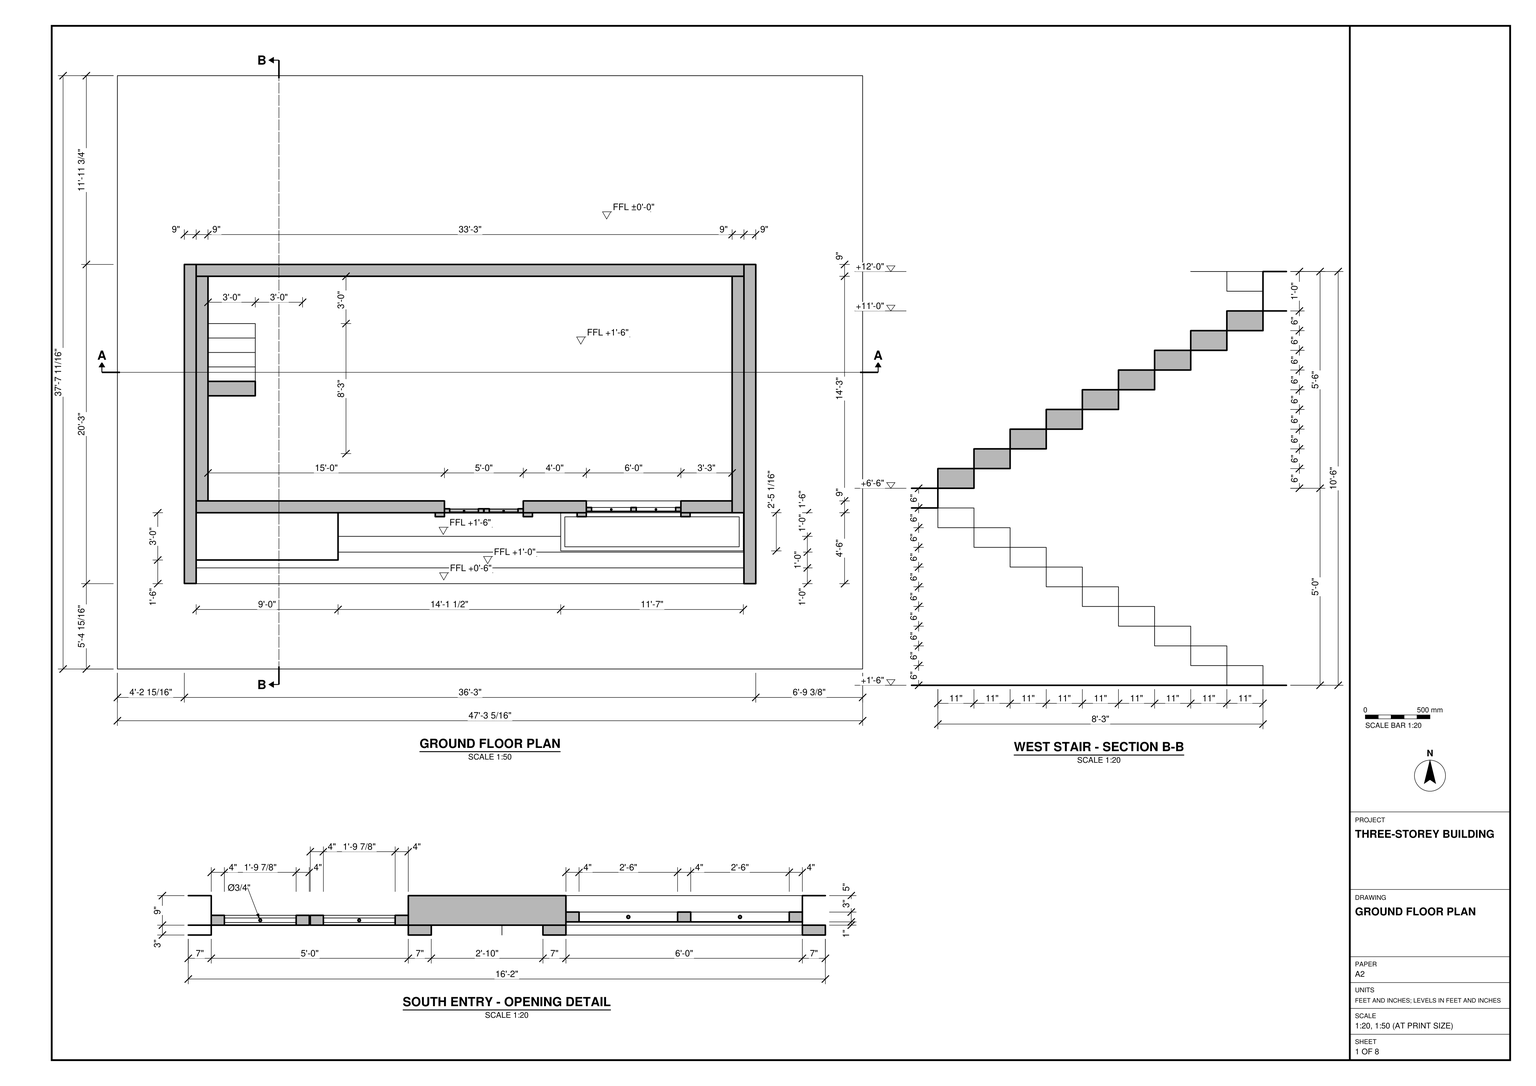
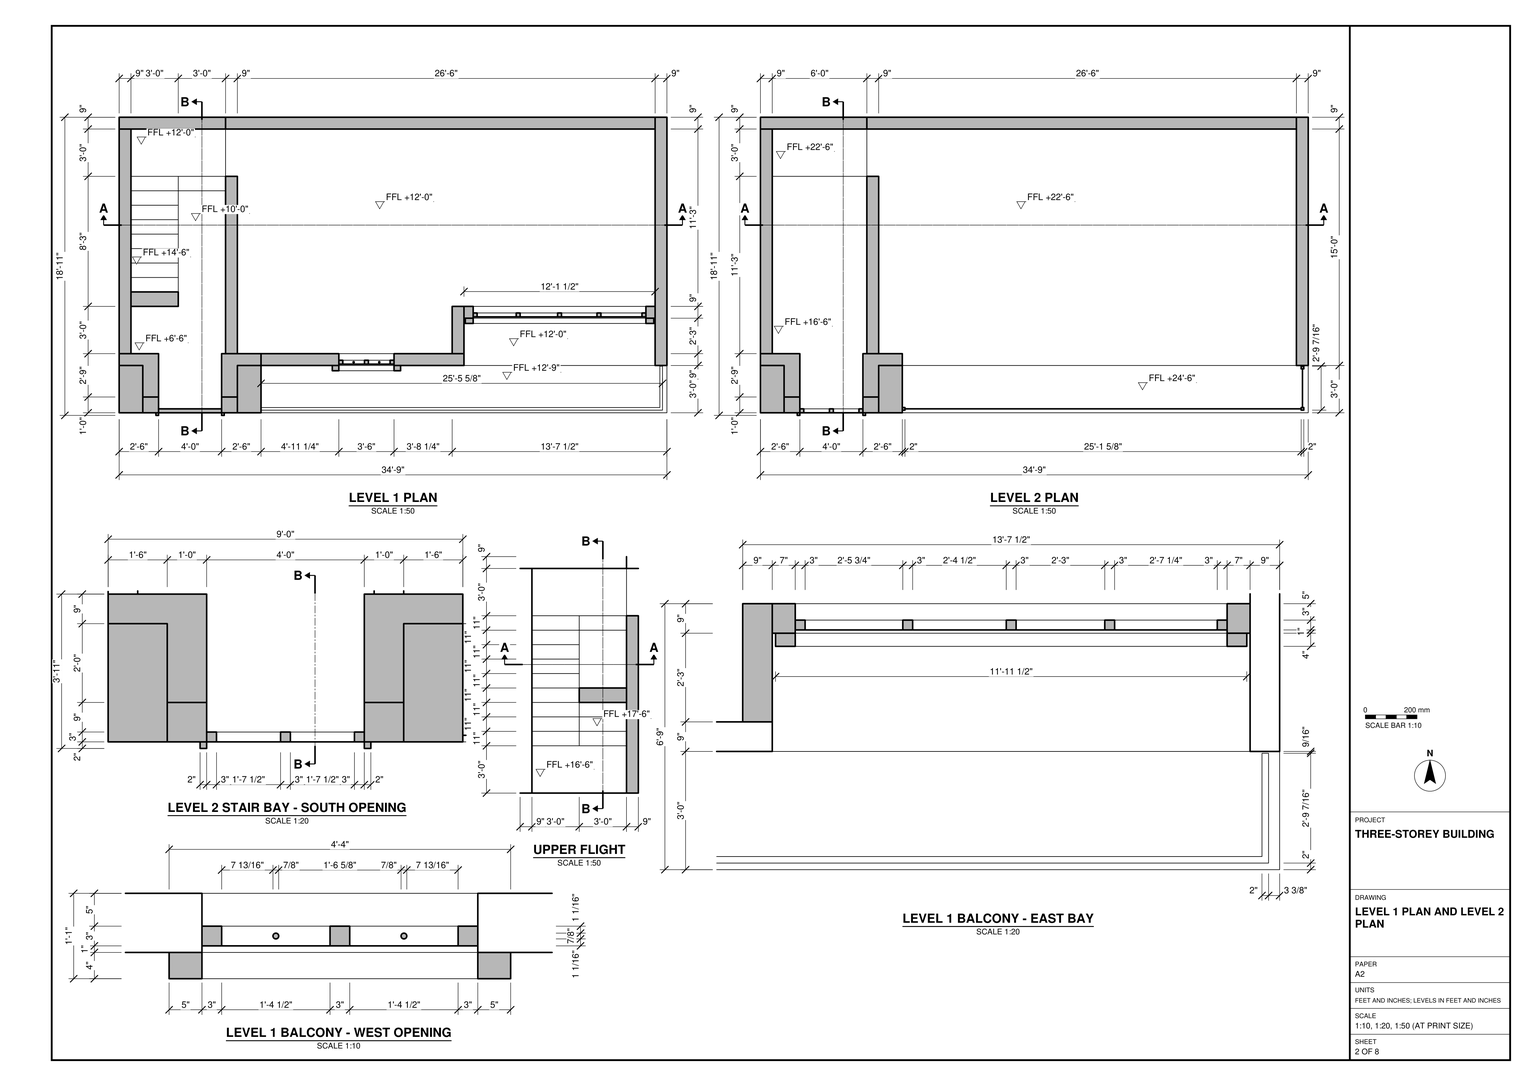
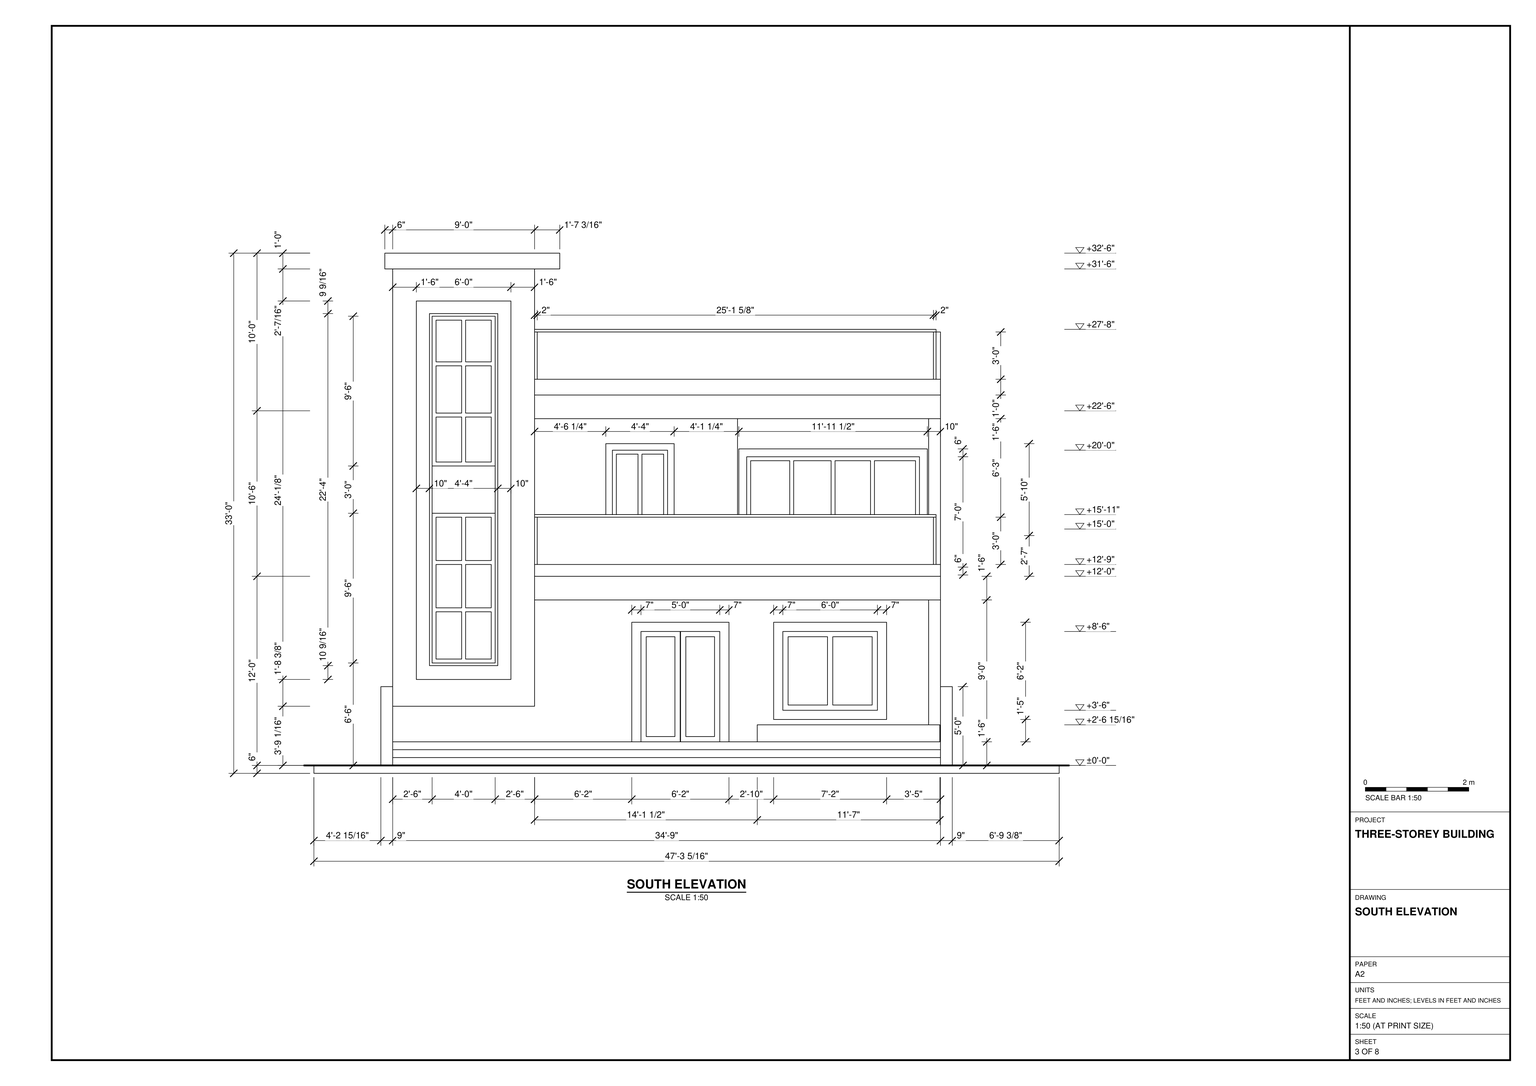
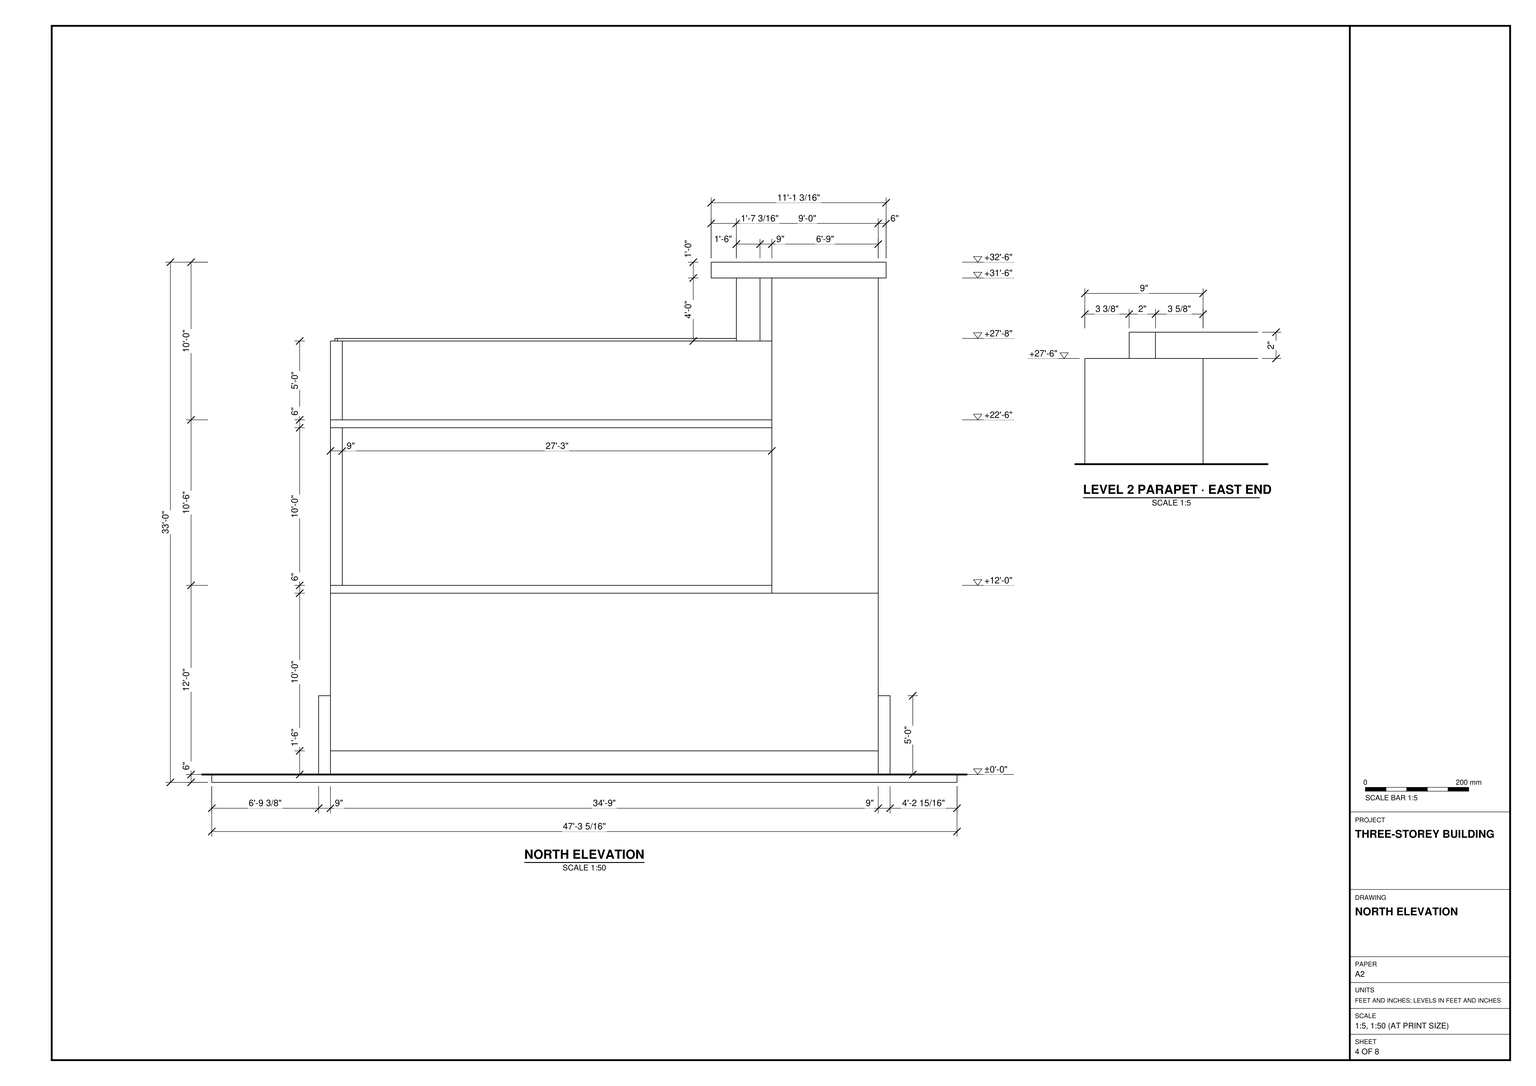
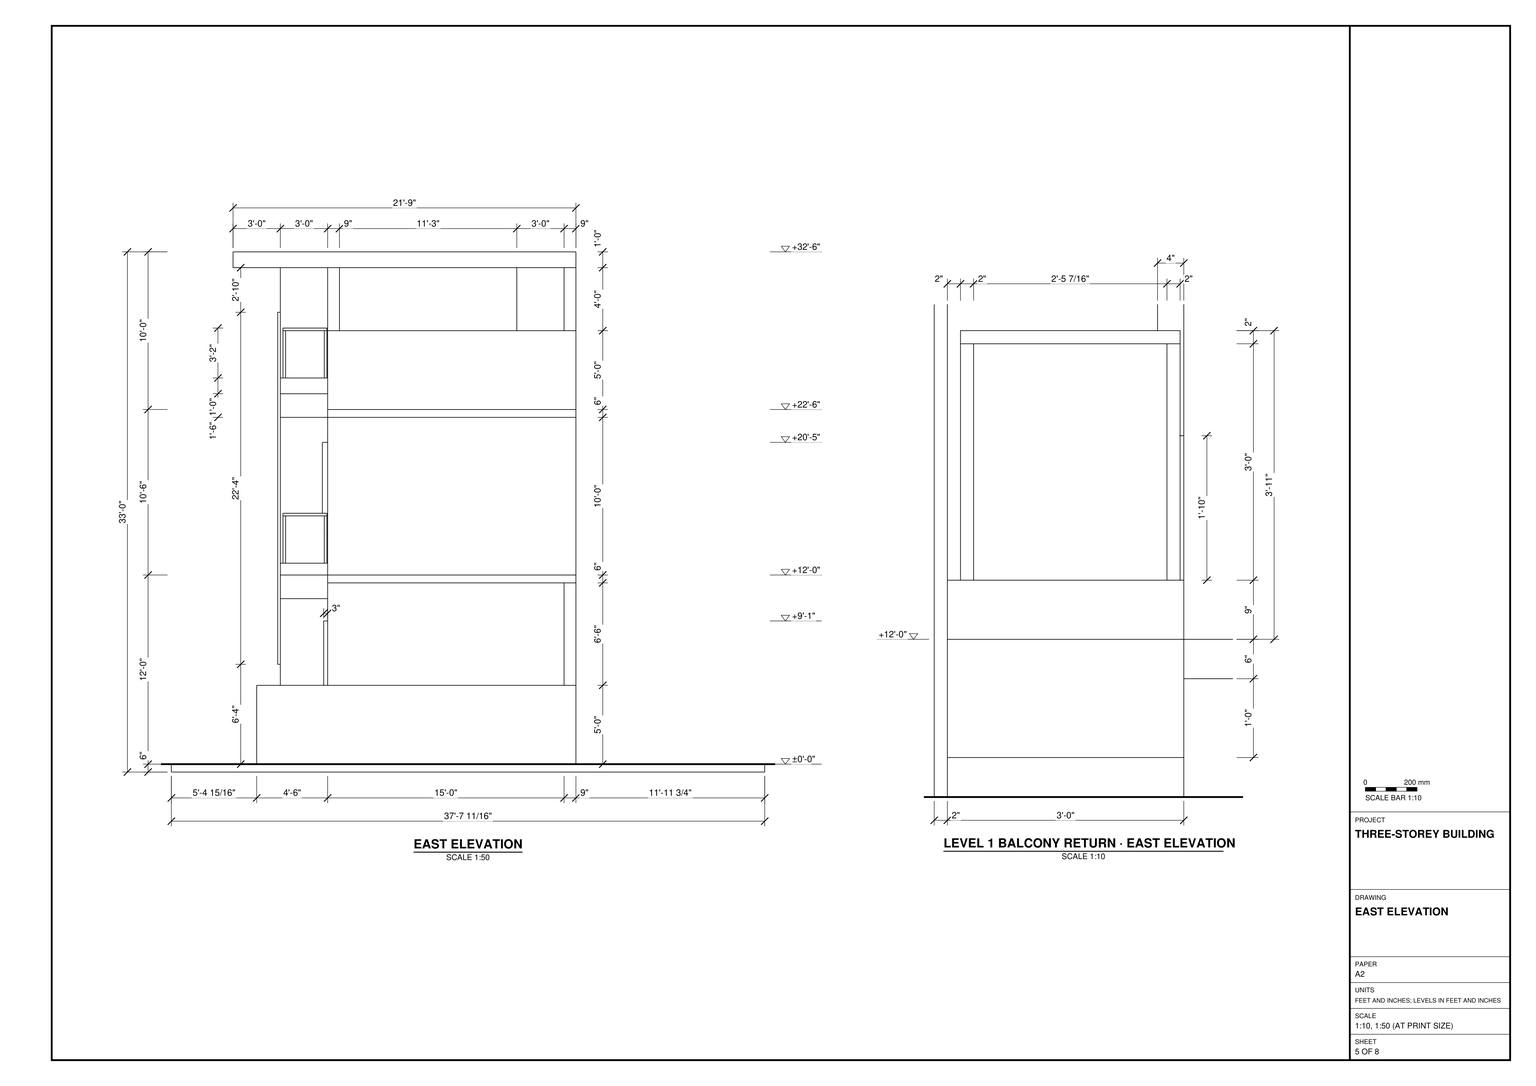
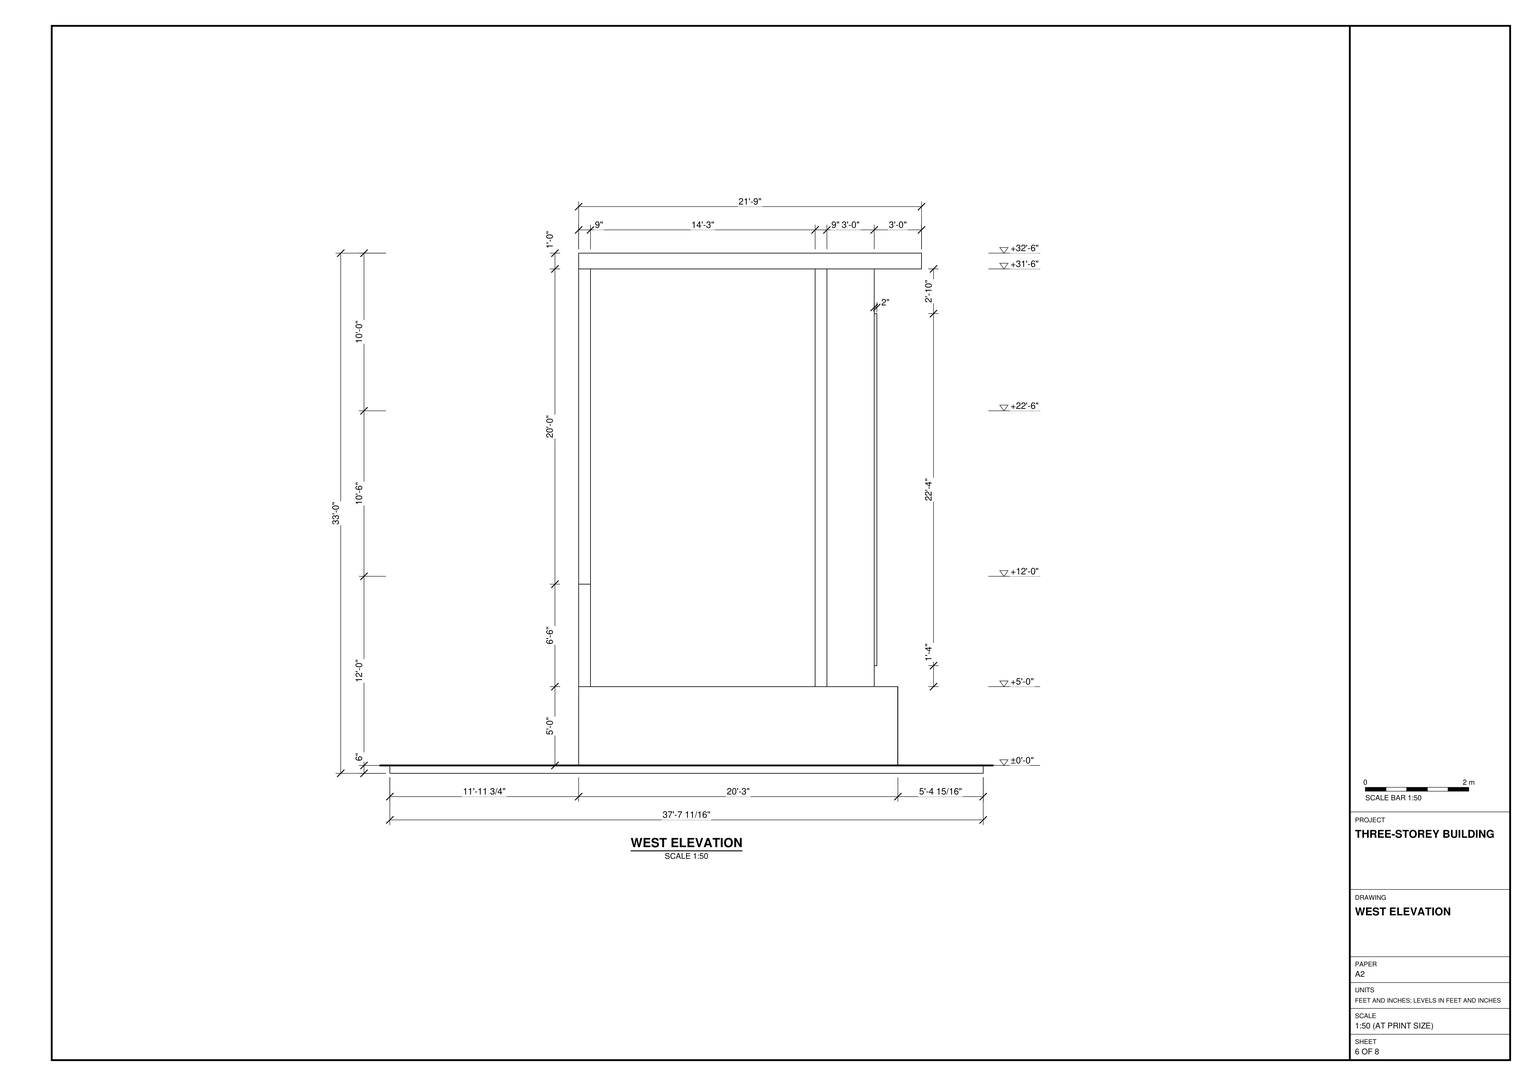
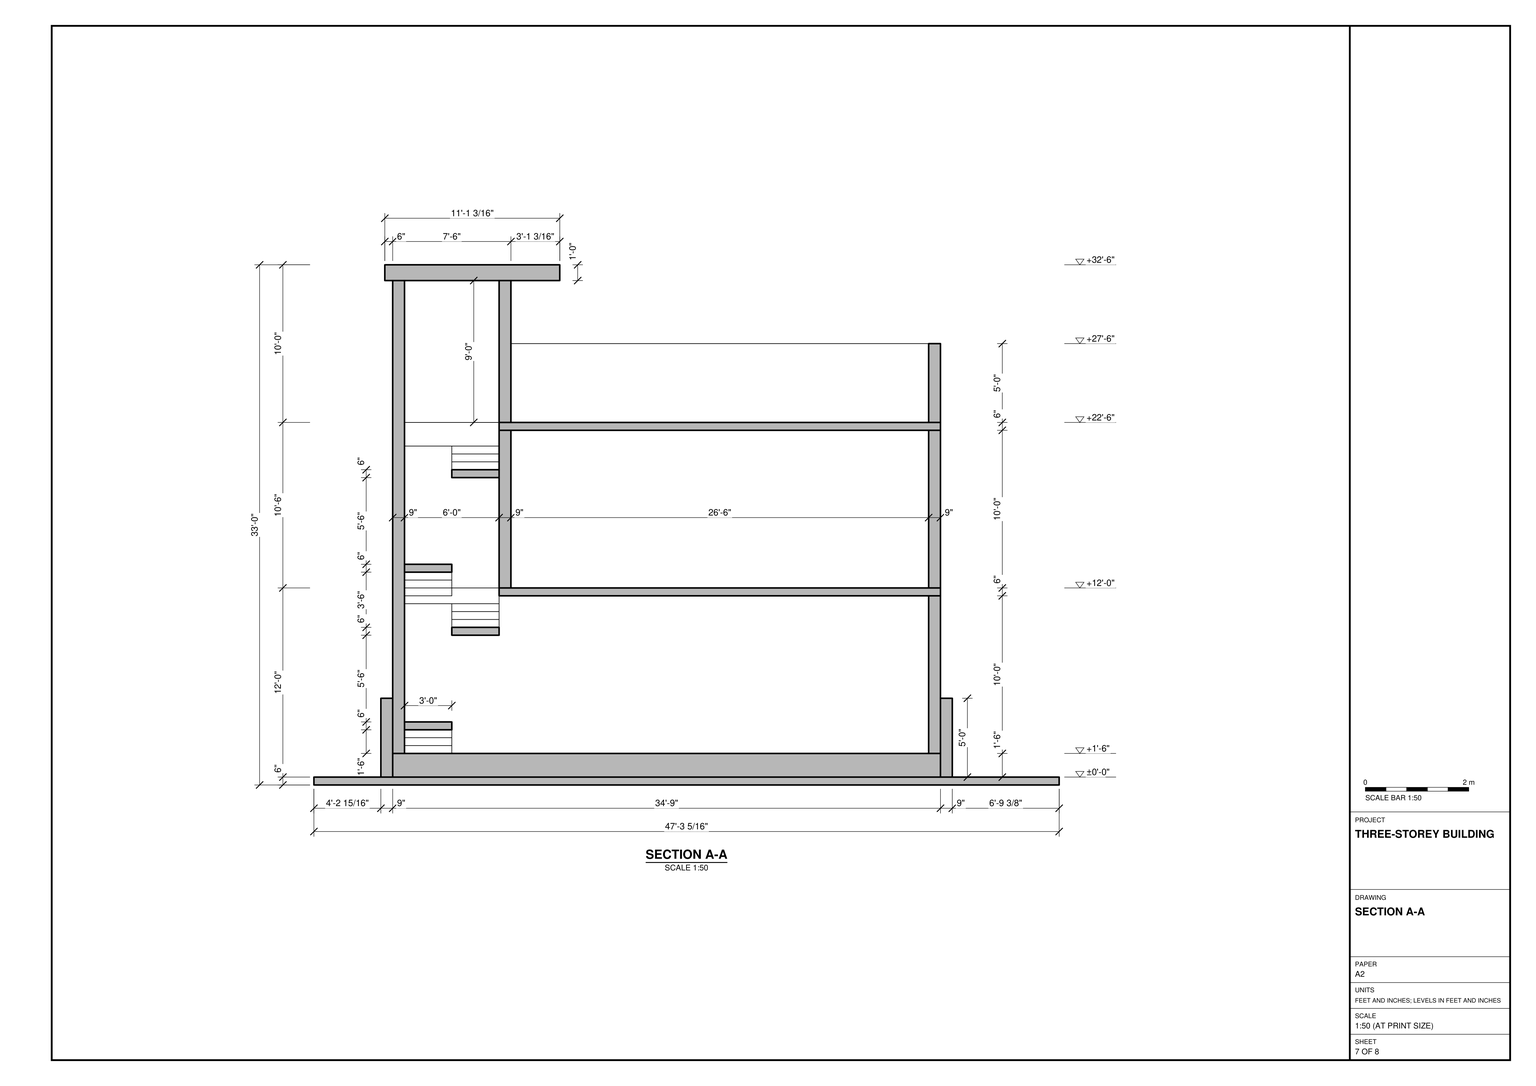
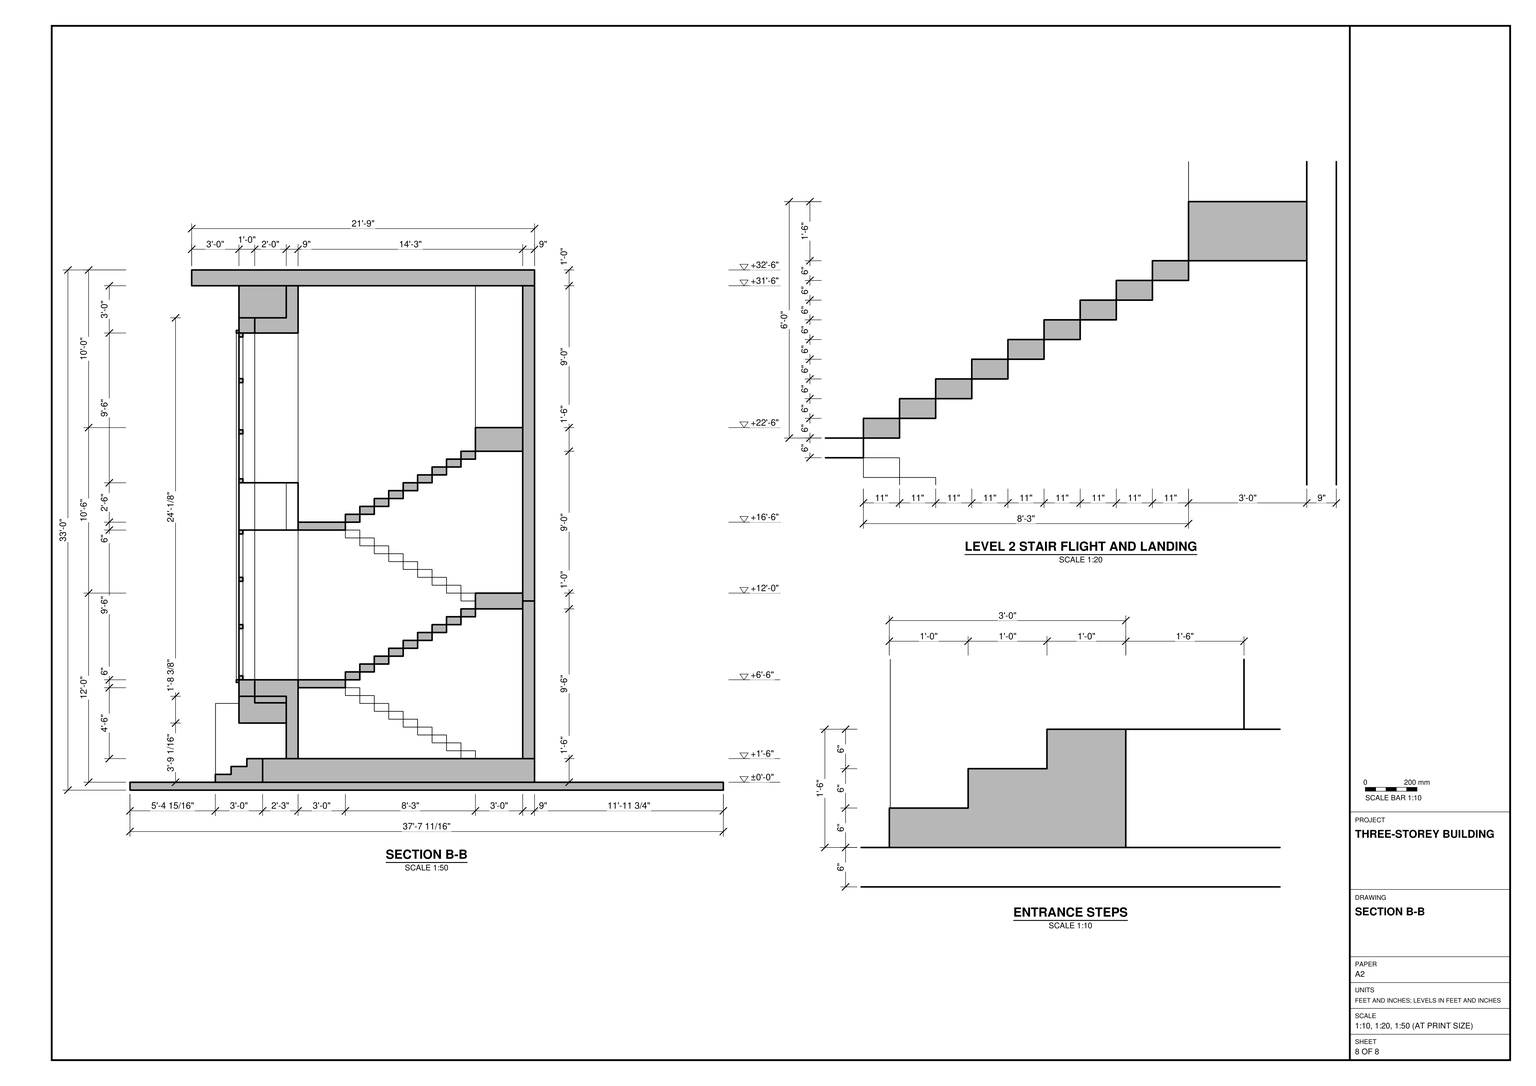
Build the three-storey building and its rectangular site base in SketchUp from task_files/diagram_01.pdf. Work in feet and inches. Including the base, the model measures 47'-3 5/16" east to west, 37'-7 11/16" north to south and 33'-0" from bottom to top. Use ±0'-0" as the ground datum, +12'-0" for Level 1 and +22'-6" for Level 2.

Locate the building on the base using the setbacks on the ground floor plan. Model the floor slabs, walls at their drawn thicknesses, and the south steps leading to the raised entry at +1'-6". Fit the paired entry door and the window to its east with the frames and pane divisions shown. At the west end, build the stair flights, intermediate landings and slab openings together so the stair connects the levels. Match the stacked glazing and projecting flat cap of the stair tower to the south elevation. Form the Level 1 balcony with its recessed east bay, and carry the upper terrace guard across the south side as drawn.

Keep shell elements such as walls, slabs and roof, and each furniture or joinery piece shown, in separate groups or components. Use components for repeated parts. Decor and loose items may be any suitable library components. Save one SketchUp model as output_files/three_storey_building_with_a_west_stair_tower.skp.

# SketchUp Ruby script. Lengths in inches.
U = 1.inch
M = Sketchup.active_model
def pt(a) = Geom::Point3d.new(a.map { |v| v * U })
def face(e, loops, mat)
  f = e.add_face(loops[0].map { |a| pt(a) })
  loops[1..].each { |l| e.add_face(l.map { |a| pt(a) }).erase! }
  f.material = f.back_material = mat if mat
  f
end
# faces: each face lists its corners as indices into pts; further lists are holes
def faces(e, pts, list, mat = nil) = list.each { |f| face(e, (f[0].is_a?(Array) ? f : [f]).map { |l| l.map { |i| pts[i] } }, mat) }
# xy, xz, yz: faces in a plane at the given z, y or x. An outline is a flat list of corners, or four numbers for a rectangle; further outlines are holes
def ring(l) = l.size == 4 ? [[l[0], l[1]], [l[2], l[1]], [l[2], l[3]], [l[0], l[3]]] : l.each_slice(2).to_a
def flat(e, list, mat, &to3) = list.each { |f| face(e, (f[0].is_a?(Array) ? f : [f]).map { |l| ring(l).map { |u, v| to3.(u, v) } }, mat) }
def xy(e, z, list, mat = nil) = flat(e, list, mat) { |x, y| [x, y, z] }
def xz(e, y, list, mat = nil) = flat(e, list, mat) { |x, z| [x, y, z] }
def yz(e, x, list, mat = nil) = flat(e, list, mat) { |y, z| [x, y, z] }
def lines(e, pts, list) = list.each { |a, b| e.add_line(pt(pts[a]), pt(pts[b])) }
# prism: a flat outline (further loops are holes) pulled along v
def prism(e, loops, v, mat = nil)
  f = face(e, loops, mat); d = Geom::Vector3d.new(v.map { |x| x * U })
  f.pushpull(f.normal.samedirection?(d) ? d.length : -d.length)
end
def box(e, o, s, mat = nil) = prism(e, [[o, [o[0] + s[0], o[1], o[2]], [o[0] + s[0], o[1] + s[1], o[2]], [o[0], o[1] + s[1], o[2]]]], [0, 0, s[2]], mat)
def at(x, y, z, deg = 0) = Geom::Transformation.translation(pt([x, y, z])) * Geom::Transformation.rotation(ORIGIN, Z_AXIS, deg.degrees)
def axes(o, x, y, z) = Geom::Transformation.new([*x, 0, *y, 0, *z, 0, *pt(o).to_a, 1])
def part(name) = M.definitions.add(name)
# library, detail: a bought-in or finely detailed component or shape, given as its bounding box
def library(name, o, s) = part(name).tap { |d| box(d.entities, o, s) }
def detail(e, o, s) = box(e.add_group.entities, o, s)
def put(e, d, t, mat = nil) = e.add_instance(d, t).tap { |i| i.material = mat if mat }
def group(e, t, mat = nil) = e.add_group.tap { |g| g.transformation = t; g.material = mat if mat }.entities
root = M.entities
M.materials.add("[Color M05]").color = [114, 114, 114]
M.materials.add("[Color M06]").color = [86, 86, 86]
M.materials.add("[Color M07]").color = [58, 58, 58]
M.materials.add("[Color M09]").color = [0, 0, 0]
M.materials.add("[Grass Dark Green]").color = [106, 157, 55]
M.materials.add("[Translucent Glass Gray]").color = [128, 128, 128]
M.materials["[Translucent Glass Gray]"].alpha = 0.5
M.materials.add("[Wood Veneer 01]").color = [120, 70, 37]
c1 = part("Group\#8")
prism(c1.entities,[[[0,0.2,0.2],[0,0.09,0.34],[0,0.02,0.51],[0,0,0.6875],[0,0.02,0.87],[0,0.09,1.03],[0,0.2,1.17],[0,0.34,1.28],[0,0.51,1.35],[0,0.6875,1.375],[0,0.87,1.35],[0,1.03,1.28],[0,1.17,1.17],[0,1.28,1.03],[0,1.35,0.87],[0,1.375,0.6875],[0,1.35,0.51],[0,1.28,0.34],[0,1.17,0.2],[0,1.03,0.09],[0,0.87,0.02],[0,0.6875,0],[0,0.51,0.02],[0,0.34,0.09]]],[25.85,0,0])
c2 = part("Group\#10")
put(c2.entities,c1,at(0,0,13.8))
put(c2.entities,c1,at(0,0,29.95))
g1 = group(c2.entities,at(10.55,0.3125,0))
prism(g1,[[[0.11,0.11,0],[0.05,0.1875,0],[0.01,0.28,0],[0,0.375,0],[0.01,0.47,0],[0.05,0.56,0],[0.11,0.64,0],[0.1875,0.7,0],[0.28,0.74,0],[0.375,0.75,0],[0.47,0.74,0],[0.56,0.7,0],[0.64,0.64,0],[0.7,0.56,0],[0.74,0.47,0],[0.75,0.375,0],[0.74,0.28,0],[0.7,0.1875,0],[0.64,0.11,0],[0.56,0.05,0],[0.47,0.01,0],[0.375,0,0],[0.28,0.01,0],[0.1875,0.05,0]]],[0,0,76])
put(c2.entities,c1,at(0,0,46.09))
put(c2.entities,c1,at(0,0,62.24))
c3 = part("Group\#15")
prism(c3.entities,[[[64,0.13,0.74],[64,0.06,0.65],[64,0.01,0.55],[64,0,0.43],[64,0.01,0.32],[64,0.06,0.22],[64,0.13,0.13],[64,0.22,0.06],[64,0.32,0.01],[64,0.43,0],[64,0.55,0.01],[64,0.65,0.06],[64,0.74,0.13],[64,0.8125,0.22],[64,0.85,0.32],[64,0.87,0.43],[64,0.85,0.55],[64,0.8125,0.65],[64,0.74,0.74],[64,0.65,0.8125],[64,0.55,0.85],[64,0.43,0.87],[64,0.32,0.85],[64,0.22,0.8125]]],[-64,0,0])
c4 = part("Group\#16")
prism(c4.entities,[[[0.01,0.55,0],[0.06,0.66,0],[0.13,0.75,0],[0.22,0.82,0],[0.32,0.86,0],[0.4375,0.875,0],[0.55,0.86,0],[0.66,0.82,0],[0.75,0.75,0],[0.82,0.66,0],[0.86,0.55,0],[0.875,0.4375,0],[0.86,0.32,0],[0.82,0.22,0],[0.75,0.13,0],[0.66,0.06,0],[0.55,0.01,0],[0.4375,0,0],[0.32,0.01,0],[0.22,0.06,0],[0.13,0.13,0],[0.06,0.22,0],[0.01,0.32,0],[0,0.4375,0]]],[0,0,52])
c5 = part("Group\#19")
box(c5.entities,[0,0,0],[36,11,6])
c6 = part("Group\#21")
put(c6.entities,c5,at(0,22,36))
put(c6.entities,c5,at(0,55,18))
put(c6.entities,c5,at(0,77,6))
put(c6.entities,c5,at(0,88,0))
put(c6.entities,c5,at(0,11,42))
put(c6.entities,c5,at(0,44,24))
put(c6.entities,c5,at(0,0,48))
put(c6.entities,c5,at(0,66,12))
put(c6.entities,c5,at(0,33,30))
c7 = part("Group\#22")
put(c7.entities,c6,at(72,135,60,180))
g2 = group(c7.entities,at(0,0,54))
box(g2,[0,0,0],[72,36,6])
put(c7.entities,c6,at(0,36,0))
c8 = part("Group\#35")
prism(c8.entities,[[[0,0.14,0.03],[0,0.08,0.0625],[0,0.04,0.11],[0,0.01,0.17],[0,0,0.23],[0,0,0.3],[0,0.03,0.36],[0,0.0625,0.42],[0,0.11,0.46],[0,0.17,0.49],[0,0.23,0.5],[0,0.3,0.49],[0,0.36,0.47],[0,0.42,0.4375],[0,0.46,0.39],[0,0.49,0.33],[0,0.5,0.26],[0,0.49,0.2],[0,0.47,0.14],[0,0.4375,0.08],[0,0.39,0.04],[0,0.33,0.01],[0,0.26,0],[0,0.2,0]]],[36,0,0])
c9 = part("Group\#36")
prism(c9.entities,[[[0.01,0.55,0],[0.06,0.66,0],[0.13,0.75,0],[0.22,0.82,0],[0.32,0.86,0],[0.4375,0.875,0],[0.55,0.86,0],[0.66,0.82,0],[0.75,0.75,0],[0.82,0.66,0],[0.86,0.55,0],[0.875,0.4375,0],[0.86,0.32,0],[0.82,0.22,0],[0.75,0.13,0],[0.66,0.06,0],[0.55,0.01,0],[0.4375,0,0],[0.32,0.01,0],[0.22,0.06,0],[0.13,0.13,0],[0.06,0.22,0],[0.01,0.32,0],[0,0.4375,0]]],[0,0,57])
c10 = part("Group\#65")
box(c10.entities,[0,2,0],[2,2,36])
c11 = part("Group\#66")
yz(c11.entities,0,[[0,0,29.4375,36]])
c12 = part("Group\#67")
xz(c12.entities,0,[[0,0,301.625,36]])
p = [[89.97,118.97,84],[89.97,118.97,348],[137.97,118.97,348],[137.97,118.97,84]]
lines(root,p,[[0,1],[1,2],[2,3],[3,0]])
g3 = group(root,at(0,92.6875,0))
box(g3,[0,-92.6875,0],[567.3125,451.6875,6])
g4 = group(root,at(56.97,118.97,6))
box(g4,[3,-18,0],[417,207,18])
g5 = group(root,at(56.97,118.97,24),"[Color M05]")
xy(g5,0,[[3,0,192,9],[252,0,411,9]])
xy(g5,24,[[300,0,372,9]])
xy(g5,42.46,[[21,-24,93,0]])
xy(g5,60,[[33,-24,81,9]])
xy(g5,84,[[192,0,252,9],[300,0,372,9]])
xy(g5,120,[[111,0,411,9]])
xy(g5,174,[[33,-36,81,9]])
xy(g5,210,[[33,-36,81,9]])
xy(g5,324,[[33,-24,81,9]])
xy(g5,335.58,[[21,-24,93,0]])
xy(g5,360,[[3,0,111,9]])
xz(g5,-36,[[33,174,81,210]])
xz(g5,-24,[[[21,42.46,93,335.58],[33,60,81,324]]])
xz(g5,0,[[[3,0,192,0,192,84,252,84,252,0,411,0,411,120,111,120,111,360,3,360],[21,42.46,93,335.58],[300,24,372,84]]])
xz(g5,9,[[[3,0,3,360,111,360,111,120,411,120,411,0,252,0,252,84,192,84,192,0],[33,210,81,324],[33,60,81,174],[300,24,372,84]]])
yz(g5,3,[[0,0,9,360]])
yz(g5,21,[[-24,42.46,0,335.58]])
yz(g5,33,[[-24,60,9,174],[-36,174,-24,210],[-24,210,9,324]])
yz(g5,81,[[-24,60,9,174],[-36,174,-24,210],[-24,210,9,324]])
yz(g5,93,[[-24,42.46,0,335.58]])
yz(g5,111,[[0,120,9,360]])
yz(g5,192,[[0,0,9,84]])
yz(g5,252,[[0,0,9,84]])
yz(g5,300,[[0,24,9,84]])
yz(g5,372,[[0,24,9,84]])
yz(g5,411,[[0,0,9,120]])
g6 = group(root,at(467.97,118.97,24))
box(g6,[0,0,0],[9,180,120])
g7 = group(root,at(241.97,115.97,24))
xy(g7,0,[[0,0,7,3],[67,0,74,3]])
xy(g7,84,[[7,0,67,3]])
xy(g7,91,[[0,0,74,3]])
xz(g7,0,[[0,0,7,0,7,84,67,84,67,0,74,0,74,91,0,91]],"[Color M06]")
xz(g7,3,[[0,0,0,91,74,91,74,0,67,0,67,84,7,84,7,0]])
yz(g7,0,[[0,0,3,91]])
yz(g7,7,[[0,0,3,84]])
yz(g7,67,[[0,0,3,84]])
yz(g7,74,[[0,0,3,91]])
p = [[67,3,0],[7,3,0]]
lines(g7,p,[[0,1]])
g8 = group(root,at(279.12,118.97,24),"[Color M06]")
prism(g8,[[[29.85,3,0],[0,3,0],[0,3,84],[29.85,3,84]],[[25.85,3,80],[4,3,80],[4,3,4],[25.85,3,4]]],[0,-3,0])
g9 = group(root,at(248.97,118.97,24),"[Color M06]")
prism(g9,[[[0,3,84],[29.85,3,84],[29.85,3,0],[0,3,0]],[[4,3,4],[25.85,3,4],[25.85,3,80],[4,3,80]]],[0,-3,0])
put(root,c2,at(252.97,119.78,28),"[Color M09]")
put(root,c2,at(283.09,119.78,28),"[Color M09]")
g10 = group(root,at(283.12,118.97,28),"[Translucent Glass Gray]")
xz(g10,0,[[0,0,21.85,76]])
g11 = group(root,at(252.97,118.97,28),"[Translucent Glass Gray]")
xz(g11,0,[[0,0,21.85,76]])
g12 = group(root,at(349.97,115.97,41))
xy(g12,0,[[0,0,86,3]])
xy(g12,7,[[7,0,79,3]])
xy(g12,67,[[7,0,79,3]])
xy(g12,74,[[0,0,86,3]])
xz(g12,0,[[[0,0,86,74],[7,7,79,67]]],"[Color M06]")
xz(g12,3,[[[0,0,86,74],[7,7,79,67]]])
yz(g12,0,[[0,0,3,74]])
yz(g12,7,[[0,7,3,67]])
yz(g12,79,[[0,7,3,67]])
yz(g12,86,[[0,0,3,74]])
g13 = group(root,at(356.97,119.97,48),"[Color M06]")
prism(g13,[[[72,3,0],[0,3,0],[0,3,60],[72,3,60]],[[34,3,4],[34,3,56],[4,3,56],[4,3,4]],[[68,3,56],[38,3,56],[38,3,4],[68,3,4]]],[0,-3,0])
put(root,c3,at(360.97,121.03,95.14),"[Color M09]")
put(root,c3,at(360.97,121.03,84.49),"[Color M09]")
put(root,c3,at(360.97,121.03,73.84),"[Color M09]")
put(root,c3,at(360.97,121.03,63.2),"[Color M09]")
put(root,c4,at(409.53,121.03,52),"[Color M09]")
put(root,c4,at(375.53,121.03,52),"[Color M09]")
g14 = group(root,at(394.97,119.97,52),"[Translucent Glass Gray]")
xz(g14,0,[[0,0,30,52]])
g15 = group(root,at(360.97,119.97,52),"[Translucent Glass Gray]")
xz(g15,0,[[0,0,30,52]])
put(root,c7,at(68.97,127.97,24))
put(root,c7,at(68.97,127.97,144))
g16 = group(root,at(56.97,298.97,24))
box(g16,[3,0,0],[417,9,120])
g17 = group(root,at(190.1,118.97,144))
prism(g17,[[[-49.13,2,0],[-49.13,189,0],[286.87,189,0],[286.87,0,0],[-22.13,0,0],[-22.13,2,0]]],[0,0,6])
g18 = group(root,at(68.97,262.97,138))
box(g18,[0,0,0],[72,36,12])
g19 = group(root,at(467.97,118.97,150))
box(g19,[0,0,0],[9,189,120])
g20 = group(root,at(167.97,298.97,150))
box(g20,[-27,0,0],[327,9,120])
g21 = group(root,at(322.47,154.97,150))
prism(g21,[[[145.5,9,0],[0,9,0],[0,9,120],[145.5,9,120]],[[7,9,91],[7,9,7],[138.5,9,7],[138.5,9,91]]],[0,-9,0])
g22 = group(root,at(329.47,155.97,157),"[Color M07]")
prism(g22,[[[0,0,0],[131.5,0,0],[131.5,0,84],[0,0,84]],[[97.25,0,81],[128.5,0,81],[128.5,0,3],[97.25,0,3]],[[32.75,0,81],[32.75,0,3],[3,0,3],[3,0,81]],[[64.25,0,3],[35.75,0,3],[35.75,0,81],[64.25,0,81]],[[94.25,0,81],[94.25,0,3],[67.25,0,3],[67.25,0,81]]],[0,3,0])
g23 = group(root,at(323.47,150.97,151))
prism(g23,[[[143.5,4,96],[143.5,4,0],[0,4,0],[0,4,96]],[[6,4,6],[137.5,4,6],[137.5,4,90],[6,4,90]]],[0,-4,0])
g24 = group(root,at(313.47,127.97,150))
box(g24,[0,0,0],[9,36,120])
g25 = group(root,at(167.97,118.97,150))
prism(g25,[[[0,0,0],[154.5,0,0],[154.5,0,120],[0,0,120]],[[59.25,0,96],[101.25,0,96],[101.25,0,36],[59.25,0,36]]],[0,9,0])
g26 = group(root,at(222.22,114.97,181))
prism(g26,[[[52,0,70],[0,0,70],[0,0,0],[52,0,0]],[[47,0,65],[47,0,5],[5,0,5],[5,0,65]]],[0,4,0])
g27 = group(root,at(227.22,119.97,186),"[Color M07]")
prism(g27,[[[0,0,60],[0,0,0],[42,0,0],[42,0,60]],[[19.5,0,57],[19.5,0,3],[3,0,3],[3,0,57]],[[22.5,0,57],[39,0,57],[39,0,3],[22.5,0,3]]],[0,3,0])
put(root,c8,at(230.22,121.22,233.18),"[Color M09]")
put(root,c8,at(230.22,121.22,222.12),"[Color M09]")
put(root,c8,at(230.22,121.22,211.06),"[Color M09]")
put(root,c8,at(230.22,121.22,200),"[Color M09]")
put(root,c9,at(238.03,121.03,189),"[Color M09]")
put(root,c9,at(257.53,121.03,189),"[Color M09]")
g28 = group(root,at(249.72,119.97,189),"[Translucent Glass Gray]")
xz(g28,0,[[0,0,16.5,54]])
g29 = group(root,at(230.22,119.97,189),"[Translucent Glass Gray]")
xz(g29,0,[[0,0,16.5,54]])
g30 = group(root,at(426.72,155.97,160),"[Translucent Glass Gray]")
xz(g30,0,[[0,0,31.25,78]])
g31 = group(root,at(396.72,155.97,160),"[Translucent Glass Gray]")
xz(g31,0,[[0,0,27,78]])
g32 = group(root,at(365.22,155.97,160),"[Translucent Glass Gray]")
xz(g32,0,[[0,0,28.5,78]])
g33 = group(root,at(332.47,155.97,160),"[Translucent Glass Gray]")
xz(g33,0,[[0,0,29.75,78]])
g34 = group(root,at(140.97,127.97,150))
box(g34,[0,0,0],[9,135,120])
g35 = group(root,at(86.97,127.97,270))
prism(g35,[[[81,0,0],[54,0,0],[54,180,0],[390,180,0],[390,-9,0],[81,-9,0]]],[0,0,6])
g36 = group(root,at(167.97,82.97,132),"[Color M06]")
xy(g36,0,[[0,0,309,36]],"[Wood Veneer 01]")
xy(g36,18,[[0,0,309,36]])
xz(g36,0,[[0,0,309,18]])
xz(g36,36,[[0,0,309,18]])
yz(g36,0,[[0,0,36,18]])
yz(g36,309,[[0,0,36,18]])
g37 = group(root,at(167.97,82.97,150))
box(g37,[0,0,0],[309,36,9])
g38 = group(root,at(89.97,82.97,84),"[Color M09]")
prism(g38,[[[0,0,114],[0,0,0],[48,0,0],[48,0,114]],[[3,0,39],[22.5,0,39],[22.5,0,3],[3,0,3]],[[45,0,39],[45,0,3],[25.5,0,3],[25.5,0,39]],[[25.5,0,78],[25.5,0,111],[45,0,111],[45,0,78]],[[22.5,0,78],[3,0,78],[3,0,111],[22.5,0,111]],[[45,0,42],[25.5,0,42],[25.5,0,75],[45,0,75]],[[3,0,42],[3,0,75],[22.5,0,75],[22.5,0,42]]],[0,3,0])
g39 = group(root,at(92.97,82.97,162),"[Translucent Glass Gray]")
xz(g39,0,[[0,0,19.5,33]])
g40 = group(root,at(115.47,82.97,162),"[Translucent Glass Gray]")
xz(g40,0,[[0,0,19.5,33]])
g41 = group(root,at(92.97,82.97,126),"[Translucent Glass Gray]")
xz(g41,0,[[0,0,19.5,33]])
g42 = group(root,at(115.47,82.97,126),"[Translucent Glass Gray]")
xz(g42,0,[[0,0,19.5,33]])
g43 = group(root,at(92.97,82.97,87),"[Translucent Glass Gray]")
xz(g43,0,[[0,0,19.5,36]])
g44 = group(root,at(115.47,82.97,87),"[Translucent Glass Gray]")
xz(g44,0,[[0,0,19.5,36]])
g45 = group(root,at(89.97,82.97,234),"[Color M09]")
prism(g45,[[[0,3,114],[48,3,114],[48,3,0],[0,3,0]],[[25.5,3,76.25],[25.5,3,40.25],[45,3,40.25],[45,3,76.25]],[[3,3,76.25],[3,3,40.25],[22.5,3,40.25],[22.5,3,76.25]],[[25.5,3,37.25],[25.5,3,3],[45,3,3],[45,3,37.25]],[[22.5,3,37.25],[3,3,37.25],[3,3,3],[22.5,3,3]],[[3,3,79.25],[22.5,3,79.25],[22.5,3,111],[3,3,111]],[[25.5,3,111],[25.5,3,79.25],[45,3,79.25],[45,3,111]]],[0,-3,0])
g46 = group(root,at(92.97,82.97,313.25),"[Translucent Glass Gray]")
xz(g46,0,[[0,0,19.5,31.75]])
g47 = group(root,at(115.47,82.97,313.25),"[Translucent Glass Gray]")
xz(g47,0,[[0,0,19.5,31.75]])
g48 = group(root,at(92.97,82.97,274.25),"[Translucent Glass Gray]")
xz(g48,0,[[0,0,19.5,36]])
g49 = group(root,at(115.47,82.97,274.25),"[Translucent Glass Gray]")
xz(g49,0,[[0,0,19.5,36]])
g50 = group(root,at(92.97,82.97,237),"[Translucent Glass Gray]")
xz(g50,0,[[0,0,19.5,34.25]])
g51 = group(root,at(115.47,82.97,237),"[Translucent Glass Gray]")
xz(g51,0,[[0,0,19.5,34.25]])
g52 = group(root,at(59.97,82.97,24))
prism(g52,[[[0,36,360],[108,36,360],[108,36,27.0625],[0,36,27.0625]],[[18,36,335.58],[18,36,47.46],[90,36,47.46],[90,36,335.58]]],[0,-36,0])
g53 = group(root,at(77.97,82.97,43.27),"[Color M05]")
prism(g53,[[[0,12,316.31],[72,12,316.31],[72,12,28.1875],[0,12,28.1875]],[[12,12,304.73],[12,12,40.73],[60,12,40.73],[60,12,304.73]]],[0,-12,0])
g54 = group(root,at(87.97,80.97,82))
prism(g54,[[[52,0,0],[52,0,268],[0,0,268],[0,0,0]],[[2,0,266],[50,0,266],[50,0,2],[2,0,2]]],[0,2,0])
put(root,c10,at(167.97,82.97,159),"[Color M09]")
put(root,c10,at(471.59,82.97,159),"[Color M09]")
put(root,c10,at(471.59,114.4,159),"[Color M09]")
put(root,c11,at(472.59,86.97,159))
put(root,c12,at(169.97,85.97,159),"[Translucent Glass Gray]")
g55 = group(root,at(167.97,82.97,270),"[Color M05]")
xy(g55,0,[[0,0,309,36]],"[Wood Veneer 01]")
xy(g55,18,[[0,0,309,36]])
xz(g55,0,[[0,0,309,18]])
xz(g55,36,[[0,0,309,18]])
yz(g55,0,[[0,0,36,18]])
yz(g55,309,[[0,0,36,18]])
g56 = group(root,at(167.97,82.97,288))
box(g56,[0,0,0],[309,36,12])
g57 = group(root,at(467.97,118.97,276))
box(g57,[0,0,0],[9,189,60])
put(root,c12,at(169.97,85.97,300),"[Translucent Glass Gray]")
put(root,c10,at(471.59,114.4,300),"[Color M09]")
put(root,c10,at(167.97,82.97,300),"[Color M09]")
put(root,c11,at(472.59,86.97,300))
put(root,c10,at(471.59,82.97,300),"[Color M09]")
g58 = group(root,at(59.97,127.97,30))
xy(g58,-6,[[0,0,9,171]])
xy(g58,228,[[9,135,81,171]])
xy(g58,246,[[9,135,81,171]])
xy(g58,354,[[0,0,9,171]])
xz(g58,0,[[0,-6,9,354]])
xz(g58,135,[[9,228,81,246]])
xz(g58,171,[[0,-6,9,354],[9,228,81,246]])
yz(g58,0,[[0,-6,171,354]])
yz(g58,9,[[0,-6,171,-6,171,228,135,228,135,354,0,354],[135,246,171,354]])
yz(g58,81,[[135,228,171,246]])
g59 = group(root,at(140.97,127.97,276))
box(g59,[0,0,0],[9,135,108])
g60 = group(root,at(56.97,298.97,144))
box(g60,[3,0,0],[81,9,240])
g61 = group(root,at(140.97,298.97,276))
box(g61,[0,0,0],[327,9,60])
g62 = group(root,at(59.97,46.97,384),"[Color M06]")
box(g62,[-6,0,0],[133.1875,261,12])
g63 = group(root,at(59.97,64.97,6))
prism(g63,[[[417,36,0],[417,36,18],[417,24,18],[417,24,12],[417,12,12],[417,12,6],[417,0,6],[417,0,0]]],[-417,0,0])
g64 = group(root,at(476.97,64.97,6))
box(g64,[0,0,0],[9,243,60])
g65 = group(root,at(50.97,65.11,6))
box(g65,[0,0,0],[9,242.85,60])
g66 = group(root,at(167.97,84.97,195),"[Color M09]")
prism(g66,[[[305.625,33.4375,0],[305.625,0,0],[0,0,0],[0,2,0],[303.625,2,0],[303.625,33.4375,0]]],[0,0,2])
g67 = group(root,at(167.97,84.97,336),"[Color M09]")
prism(g67,[[[305.625,0,0],[0,0,0],[0,2,0],[303.625,2,0],[303.625,33.4375,0],[305.625,33.4375,0]]],[0,0,2])
g68 = group(root,at(337.48,89.9,24),"[Color M05]")
xy(g68,0,[[0,0,139,29.0625]])
xy(g68,12.4375,[[3.13,3.13,135.87,25.93]],"[Grass Dark Green]")
xy(g68,12.9375,[[[0,0,139,29.0625],[3.13,3.13,135.87,25.93]]])
xz(g68,0,[[0,0,139,12.9375]])
xz(g68,3.13,[[3.13,12.4375,135.87,12.9375]])
xz(g68,25.93,[[3.13,12.4375,135.87,12.9375]])
xz(g68,29.0625,[[0,0,139,12.9375]])
yz(g68,0,[[0,0,29.0625,12.9375]])
yz(g68,3.13,[[3.13,12.4375,25.93,12.9375]])
yz(g68,135.87,[[3.13,12.4375,25.93,12.9375]])
yz(g68,139,[[0,0,29.0625,12.9375]])
